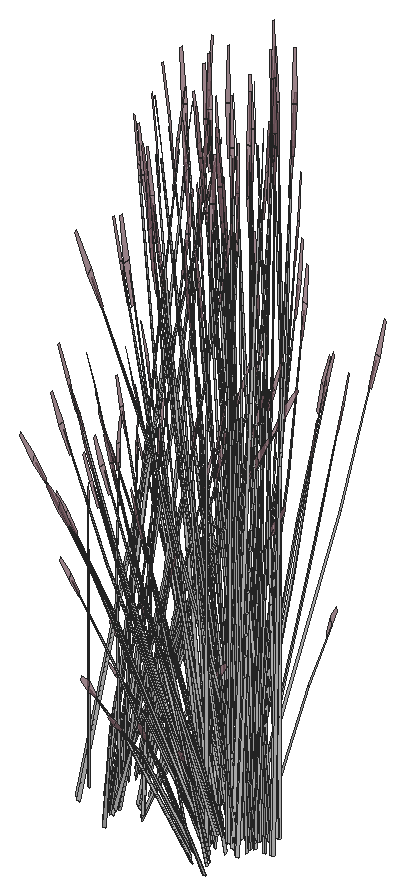
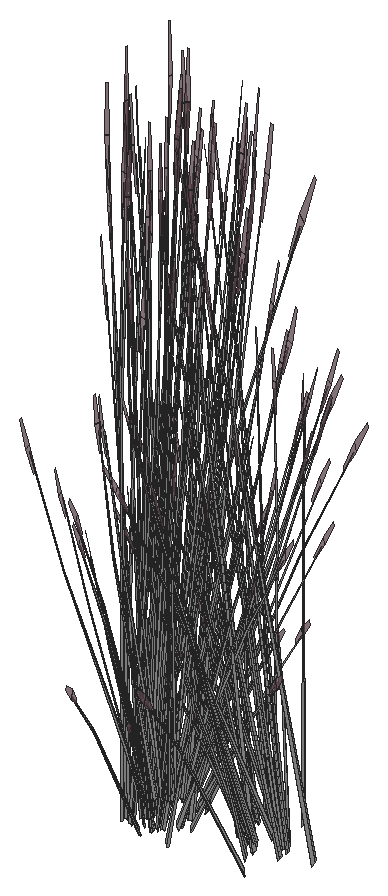
# SketchUp Ruby script. Lengths in inches.
U = 1.inch
M = Sketchup.active_model
def pt(a) = Geom::Point3d.new(a.map { |v| v * U })
def face(e, loops, mat)
  f = e.add_face(loops[0].map { |a| pt(a) })
  loops[1..].each { |l| e.add_face(l.map { |a| pt(a) }).erase! }
  f.material = f.back_material = mat if mat
  f
end
# faces: each face lists its corners as indices into pts; further lists are holes
def faces(e, pts, list, mat = nil) = list.each { |f| face(e, (f[0].is_a?(Array) ? f : [f]).map { |l| l.map { |i| pts[i] } }, mat) }
# xy, xz, yz: faces in a plane at the given z, y or x. An outline is a flat list of corners, or four numbers for a rectangle; further outlines are holes
def ring(l) = l.size == 4 ? [[l[0], l[1]], [l[2], l[1]], [l[2], l[3]], [l[0], l[3]]] : l.each_slice(2).to_a
def flat(e, list, mat, &to3) = list.each { |f| face(e, (f[0].is_a?(Array) ? f : [f]).map { |l| ring(l).map { |u, v| to3.(u, v) } }, mat) }
def xy(e, z, list, mat = nil) = flat(e, list, mat) { |x, y| [x, y, z] }
def xz(e, y, list, mat = nil) = flat(e, list, mat) { |x, z| [x, y, z] }
def yz(e, x, list, mat = nil) = flat(e, list, mat) { |y, z| [x, y, z] }
def lines(e, pts, list) = list.each { |a, b| e.add_line(pt(pts[a]), pt(pts[b])) }
# prism: a flat outline (further loops are holes) pulled along v
def prism(e, loops, v, mat = nil)
  f = face(e, loops, mat); d = Geom::Vector3d.new(v.map { |x| x * U })
  f.pushpull(f.normal.samedirection?(d) ? d.length : -d.length)
end
def box(e, o, s, mat = nil) = prism(e, [[o, [o[0] + s[0], o[1], o[2]], [o[0] + s[0], o[1] + s[1], o[2]], [o[0], o[1] + s[1], o[2]]]], [0, 0, s[2]], mat)
def at(x, y, z, deg = 0) = Geom::Transformation.translation(pt([x, y, z])) * Geom::Transformation.rotation(ORIGIN, Z_AXIS, deg.degrees)
def axes(o, x, y, z) = Geom::Transformation.new([*x, 0, *y, 0, *z, 0, *pt(o).to_a, 1])
def part(name) = M.definitions.add(name)
# library, detail: a bought-in or finely detailed component or shape, given as its bounding box
def library(name, o, s) = part(name).tap { |d| box(d.entities, o, s) }
def detail(e, o, s) = box(e.add_group.entities, o, s)
def put(e, d, t, mat = nil) = e.add_instance(d, t).tap { |i| i.material = mat if mat }
def group(e, t, mat = nil) = e.add_group.tap { |g| g.transformation = t; g.material = mat if mat }.entities
root = M.entities
M.materials.add("LightPink_Translucent").color = [144, 107, 117]
M.materials["LightPink_Translucent"].alpha = 0.75
M.materials.add("[_0053_Ivory_]").color = [200, 200, 200]
c1 = part("blade")
p = [[2.15,0.21,22],[0,0.17,0],[0.09,0.45,0],[2.18,0.31,22],[2.29,0.31,22],[0.38,0.45,0],
  [2.48,0.24,33],[2.49,0.24,33],[2.48,0.22,33]]
faces(c1.entities,p,[[0,1,2,3],[4,5,2,3],[6,3,4,7],[8,0,3,6]])
c2 = part("seeds")
p = [[0.3,-0.1,1.38],[-0.01,-0.03,1.59],[-0.01,-0.03,0.03],[0.14,-0.07,-0.07],[0.29,-0.03,3],[0.15,0.01,3.11]]
faces(c2.entities,p,[[0,1,2,3],[1,0,4,5]],"LightPink_Translucent")
c3 = part("blade with seeds")
put(c3.entities,c1,at(0,0,0))
put(c3.entities,c2,axes([2.4,0.25,30.99],[1.5799,-0.05474,1.17369],[-0.12525,1.92788,0.29478],[-0.07173,-0.02425,1.56792]))
put(root,c3,axes([430.06,98.57,130.53],[0.21074,-0.13302,1.71376],[0.17741,0.61464,0.13857],[-0.33083,0.13891,0.73262]),"[_0053_Ivory_]")
put(root,c3,axes([429.4,99.62,129.24],[0.21107,0.05162,1.43002],[0.13604,0.52729,-0.30754],[-0.28671,0.0987,0.61141]),"[_0053_Ivory_]")
put(root,c3,axes([422.4,96.86,128.68],[0.14267,0.54795,-0.30978],[-0.56663,0.1556,0.30978],[0.11423,0.06319,1.38974]),"[_0053_Ivory_]")
put(root,c3,axes([423.47,98.64,129.03],[0.75945,0,0],[0,0.70283,-0.51607],[0,0.16007,1.63711]),"[_0053_Ivory_]")
put(root,c3,axes([421.01,97.73,129.32],[0.61322,-0.4175,-0.29095],[0.40778,0.58992,-0.50002],[0.1513,0.05991,1.59708]),"[_0053_Ivory_]")
put(root,c3,axes([431.27,97.93,130],[0.17264,-0.09097,1.77064],[0.05953,0.63516,0.13857],[-0.37394,0.08428,0.63284]),"[_0053_Ivory_]")
put(root,c3,axes([422.49,101.25,129.32],[-0.38947,-0.01972,1.0506],[0.25721,-0.41888,0.58006],[0.15386,0.14882,0.8241]),"[_0053_Ivory_]")
put(root,c3,axes([421.3125,96.22,130.53],[-0.11309,0.21615,1.71376],[-0.47441,-0.44731,0.13857],[0.21402,-0.27879,0.73262]),"[_0053_Ivory_]")
put(root,c3,axes([430.71,96.91,131.63],[-0.60713,-0.01514,-0.71045],[0.04078,-0.63759,0.08574],[-0.25721,-0.06729,1.00501]),"[_0053_Ivory_]")
put(root,c3,axes([419.47,97.36,128.25],[-0.59782,0.25177,1.28929],[-0.19028,-0.72239,0.50096],[0.36709,0.01202,1.46642]),"[_0053_Ivory_]")
put(root,c3,axes([430.22,97.07,129.24],[0.11858,0.17508,1.43002],[-0.27325,0.4759,-0.30754],[-0.28057,-0.11375,0.61141]),"[_0053_Ivory_]")
put(root,c3,axes([429.73,98.02,131.18],[-0.50475,-0.17543,-0.35414],[0.14722,-0.5118,0.4572],[-0.20322,0.04693,0.87481]),"[_0053_Ivory_]")
put(root,c3,axes([430.43,96.5,130.53],[0.2256,0.10835,1.71376],[-0.46687,0.45453,0.13857],[-0.29098,-0.20505,0.73262]),"[_0053_Ivory_]")
put(root,c3,axes([421.66,100.67,131.33],[0.59932,-0.14948,-0.51099],[0.10484,0.56611,-0.3958],[0.16097,0.16223,0.97773]),"[_0053_Ivory_]")
put(root,c3,axes([422.21,96.24,129.03],[0.37973,-0.63014,0],[0.6353,0.35142,-0.51607],[0.14469,0.08004,1.63711]),"[_0053_Ivory_]")
put(root,c3,axes([422.85,95.97,128.15],[-0.0909,-0.04954,1.76342],[-0.2335,-0.55347,-0.26939],[0.15752,-0.1502,0.30037]),"[_0053_Ivory_]")
put(root,c3,axes([430.08,98.28,131.33],[-0.16454,0.57202,-0.51099],[-0.56413,-0.19607,-0.3958],[-0.22713,0.05245,0.97773]),"[_0053_Ivory_]")
put(root,c3,axes([422.56,96.62,128.67],[0.56842,0.31443,-0.49651],[-0.33976,0.56381,0],[0.12946,0.07161,1.57504]),"[_0053_Ivory_]")
put(root,c3,axes([430.51,97.04,131.33],[-0.44101,0.41656,-0.51099],[-0.38623,-0.44004,-0.3958],[-0.22407,-0.06338,0.97773]),"[_0053_Ivory_]")
put(root,c3,axes([429.8,98.24,128.15],[0.0154,0.09911,1.76342],[-0.31051,0.51756,-0.26939],[-0.22056,-0.02609,0.30037]),"[_0053_Ivory_]")
put(root,c3,axes([422.53,101.1,128.15],[0.04425,-0.09079,1.76342],[0.55709,-0.26738,-0.26939],[0.16889,0.13839,0.30037]),"[_0053_Ivory_]")
put(root,c3,axes([422.83,97.3,131.33],[-0.15602,-0.5742,-0.51099],[0.59087,-0.10045,-0.3958],[0.16933,-0.15423,0.97773]),"[_0053_Ivory_]")
put(root,c3,axes([423.87,100.26,130.58],[-0.11624,-0.52862,-0.03492],[0.54943,-0.12153,-0.15832],[0.11473,0.03351,0.52218]),"[_0053_Ivory_]")
put(root,c3,axes([421.73,97.83,128.71],[0.63179,0.1031,-0.62353],[-0.13332,0.63596,-0.16365],[0.18854,0.07706,1.37633]),"[_0053_Ivory_]")
put(root,c3,axes([428.96,100.73,129.42],[0.25312,-0.28501,1.1486],[0.09988,0.45119,0.84392],[-0.18292,0.08079,0.25299]),"[_0053_Ivory_]")
put(root,c3,axes([424.42,98.2,128.91],[-0.37654,-0.40212,-0.06488],[0.4124,-0.36845,-0.29416],[0.11685,-0.02594,0.97024]),"[_0053_Ivory_]")
put(root,c3,axes([423.56,96.15,129.42],[-0.2023,0.32011,1.1486],[-0.17388,-0.43009,0.84392],[0.16708,-0.10777,0.25299]),"[_0053_Ivory_]")
put(root,c3,axes([430.34,96.65,131.18],[-0.34557,-0.39372,-0.35414],[0.39459,-0.37271,0.4572],[-0.20048,-0.05671,0.87481]),"[_0053_Ivory_]")
put(root,c3,axes([430.83,98.99,130.53],[0.1517,-0.19322,1.71376],[0.38303,0.52154,0.13857],[-0.26271,0.23751,0.73262]),"[_0053_Ivory_]")
put(root,c3,axes([429.92,99.49,131.18],[-0.52868,0.08987,-0.35414],[-0.1396,-0.51376,0.4572],[-0.1515,0.13799,0.87481]),"[_0053_Ivory_]")
put(root,c3,axes([429.63,101.02,128.15],[0.08147,0.06283,1.76342],[0.13814,0.58211,-0.26939],[-0.18056,0.12413,0.30037]),"[_0053_Ivory_]")
put(root,c3,axes([429.51,97.59,129.42],[0.38775,-0.045,1.1486],[-0.24596,0.39648,0.84392],[-0.19161,-0.05948,0.25299]),"[_0053_Ivory_]")
put(root,c3,axes([421.6,99.19,130.53],[-0.2256,-0.10835,1.71376],[0.46687,-0.45453,0.13857],[0.29098,0.20505,0.73262]),"[_0053_Ivory_]")
put(root,c3,axes([423.27,97.36,131.18],[0.52868,-0.08987,-0.35414],[0.1396,0.51376,0.4572],[0.1515,-0.13799,0.87481]),"[_0053_Ivory_]")
put(root,c3,axes([422.85,97.53,131.63],[0.31725,-0.49618,-0.71045],[0.55593,0.35263,0.08574],[0.18942,-0.17977,1.00501]),"[_0053_Ivory_]")
put(root,c3,axes([422.84,100.2,131.18],[0.34557,0.39372,-0.35414],[-0.39459,0.37271,0.4572],[0.20048,0.05671,0.87481]),"[_0053_Ivory_]")
put(root,c3,axes([430.72,99.46,130.53],[0.11309,-0.21615,1.71376],[0.47441,0.44731,0.13857],[-0.21402,0.27879,0.73262]),"[_0053_Ivory_]")
put(root,c3,axes([430.35,99.55,131.33],[0.15602,0.5742,-0.51099],[-0.59087,0.10045,-0.3958],[-0.16933,0.15423,0.97773]),"[_0053_Ivory_]")
put(root,c3,axes([431.83,99.14,128.71],[-0.63179,-0.1031,-0.62353],[0.13332,-0.63596,-0.16365],[-0.18854,-0.07706,1.37633]),"[_0053_Ivory_]")
put(root,c3,axes([423.11,98.57,131.33],[0.16454,-0.57202,-0.51099],[0.56413,0.19607,-0.3958],[0.22713,-0.05245,0.97773]),"[_0053_Ivory_]")
put(root,c3,axes([424.52,98.9375,129.42],[-0.37526,0.10382,1.1486],[0.17664,-0.42906,0.84392],[0.19907,0.02936,0.25299]),"[_0053_Ivory_]")
put(root,c3,axes([431.76,96.16,131.63],[-0.51789,-0.30395,-0.71045],[0.36805,-0.53263,0.08574],[-0.18764,-0.18149,1.00501]),"[_0053_Ivory_]")
put(root,c3,axes([431.52,96.18,131.33],[-0.59932,0.14948,-0.51099],[-0.10484,-0.56611,-0.3958],[-0.16097,-0.16223,0.97773]),"[_0053_Ivory_]")
put(root,c3,axes([423.31,97.07,129.24],[-0.21697,-0.01863,1.43002],[-0.22228,-0.49966,-0.30754],[0.26655,-0.14135,0.61141]),"[_0053_Ivory_]")
put(root,c3,axes([423.45,98.83,131.18],[0.50475,0.17543,-0.35414],[-0.14722,0.5118,0.4572],[0.20322,-0.04693,0.87481]),"[_0053_Ivory_]")
put(root,c3,axes([431,100.34,128.67],[-0.56842,-0.31443,-0.49651],[0.33976,-0.56381,0],[-0.12946,-0.07161,1.57504]),"[_0053_Ivory_]")
put(root,c3,axes([430.75,95.66,128.15],[-0.05883,0.08284,1.76342],[-0.59454,0.17861,-0.26939],[-0.14363,-0.16248,0.30037]),"[_0053_Ivory_]")
put(root,c3,axes([422.48,99.9375,131.63],[0.60713,0.01514,-0.71045],[-0.04078,0.63759,0.08574],[0.25721,0.06729,1.00501]),"[_0053_Ivory_]")
put(root,c3,axes([431.34,100.72,129.03],[-0.37973,0.63014,0],[-0.6353,-0.35142,-0.51607],[-0.14469,-0.08004,1.63711]),"[_0053_Ivory_]")
put(root,c3,axes([423.71,98.73,128.64],[-0.39118,0.07547,1.41583],[-0.06226,-0.6007,0.08104],[0.27398,-0.09092,0.80566]),"[_0053_Ivory_]")
put(root,c3,axes([424.14,98.34,128.15],[-0.03174,-0.09547,1.76342],[0.22015,-0.55846,-0.26939],[0.22208,-0.00803,0.30037]),"[_0053_Ivory_]")
put(root,c3,axes([422.08,98.2,130.53],[-0.25192,0.01424,1.71376],[0.16712,-0.61729,0.13857],[0.35901,0.03818,0.73262]),"[_0053_Ivory_]")
put(root,c3,axes([430.65,101.64,129.24],[0.19166,-0.0992,1.43002],[0.4732,0.29912,-0.30754],[-0.14084,0.25882,0.61141]),"[_0053_Ivory_]")
put(root,c3,axes([423,98.78,131.63],[0.53369,-0.27773,-0.71045],[0.29743,0.5717,0.08574],[0.25786,-0.06494,1.00501]),"[_0053_Ivory_]")
put(root,c3,axes([430.38,95.98,128.78],[-0.1752,0.51349,-0.03893],[-0.53924,-0.15795,-0.17649],[-0.08187,-0.08399,0.58215]),"[_0053_Ivory_]")
put(root,c3,axes([431.18,95.33,129.24],[-0.03678,0.20572,1.43002],[-0.53767,0.17221,-0.30754],[-0.12568,-0.26589,0.61141]),"[_0053_Ivory_]")
put(root,c3,axes([431.36,95.87,130.53],[0.13883,0.2019,1.71376],[-0.64153,0.16998,0.13857],[-0.14499,-0.31697,0.73262]),"[_0053_Ivory_]")
put(root,c3,axes([432.54,99.24,129.32],[-0.61322,0.4175,-0.29095],[-0.40778,-0.58992,-0.50002],[-0.1513,-0.05991,1.59708]),"[_0053_Ivory_]")
put(root,c3,axes([431.58,95.76,131.18],[-0.0938,-0.50652,-0.35414],[0.53623,-0.13375,0.4572],[-0.14403,-0.14515,0.87481]),"[_0053_Ivory_]")
put(root,c3,axes([430.09,98.32,129.03],[-0.75945,0,0],[0,-0.70283,-0.51607],[0,-0.16007,1.63711]),"[_0053_Ivory_]")
put(root,c3,axes([431.16,100.11,128.68],[-0.14267,-0.54795,-0.30978],[0.56663,-0.1556,0.30978],[-0.11423,-0.06319,1.38974]),"[_0053_Ivory_]")
put(root,c3,axes([423.82,99.625,129.24],[-0.14627,-0.15466,1.43002],[0.19032,-0.51164,-0.30754],[0.29594,0.06931,0.61141]),"[_0053_Ivory_]")
put(root,c3,axes([430.85,100.68,131.18],[-0.41095,0.33109,-0.35414],[-0.38901,-0.37805,0.4572],[-0.05919,0.19208,0.87481]),"[_0053_Ivory_]")
put(root,c3,axes([432.95,99.69,128.71],[-0.40909,0.47266,-0.62353],[-0.50819,-0.4286,-0.16365],[-0.16393,0.11791,1.37633]),"[_0053_Ivory_]")
put(root,c3,axes([430.68,98.14,128.98],[-0.56493,0.5287,0.30756],[-0.56528,-0.52313,-0.36492],[-0.01973,-0.15014,1.64885]),"[_0053_Ivory_]")
put(root,c3,axes([433,99.6,129.98],[0.52485,0.25358,1.51261],[-0.51417,0.54629,0.59816],[-0.23031,-0.32378,1.26806]),"[_0053_Ivory_]")
put(root,c3,axes([431,95,129.42],[0.31682,0.21887,1.1486],[-0.4614,0.13157,0.84392],[-0.09872,-0.16821,0.25299]),"[_0053_Ivory_]")
put(root,c3,axes([433.23,99.43,129.12],[-0.59306,-0.50614,-0.25192],[0.49904,-0.56836,0.5513],[-0.1597,0.05921,1.68216]),"[_0053_Ivory_]")
put(root,c3,axes([432.15,98.9375,128.86],[-0.36485,-0.52782,-0.44739],[0.55265,-0.37168,0.21531],[-0.11807,-0.06531,1.43643]),"[_0053_Ivory_]")
put(root,c3,axes([431.12,100.33,131.99],[-0.0158,0.58168,-0.7886],[-0.66548,-0.03907,0.09517],[-0.07023,0.24643,1.11556]),"[_0053_Ivory_]")
put(root,c3,axes([431.11,101.97,129.42],[-0.01572,-0.37392,1.1486],[0.39276,0.26669,0.84392],[-0.07724,0.17822,0.25299]),"[_0053_Ivory_]")
put(root,c3,axes([432.93,99.32,128.86],[-0.65953,0.03882,-0.44739],[-0.05964,-0.64439,0.21531],[-0.11807,0.06531,1.43643]),"[_0053_Ivory_]")
put(root,c3,axes([431.67,100.4,129.13],[0.56842,0.31443,0.49651],[-0.33976,0.56381,0],[-0.12946,-0.07161,1.57504]),"[_0053_Ivory_]")
put(root,c3,axes([430.9,101.15,130.02],[0.01334,-0.32463,1.54345],[0.60018,0.17147,0.21329],[-0.052,0.34598,0.72882]),"[_0053_Ivory_]")
put(root,c3,axes([432.21,99.24,129.09],[0.16098,-0.74515,-0.23429],[0.76326,0.12989,0.51271],[-0.13337,-0.1029,1.5644]),"[_0053_Ivory_]")
put(root,c3,axes([432.49,99.42,129.27],[-0.11717,0.56122,0.1448],[-0.57245,-0.09742,-0.41347],[-0.10418,-0.05763,1.26744]),"[_0053_Ivory_]")
put(root,c3,axes([433.625,100.98,128.67],[-0.56842,0.31443,-0.49651],[-0.33976,-0.56381,0],[-0.12946,0.07161,1.57504]),"[_0053_Ivory_]")
put(root,c3,axes([430.26,97.85,128.67],[0,-0.62885,-0.49651],[0.67951,0,0],[0,-0.14322,1.57504]),"[_0053_Ivory_]")
put(root,c3,axes([430.55,98.43,129.13],[0,0.62885,0.49651],[-0.67951,0,0],[0,-0.14322,1.57504]),"[_0053_Ivory_]")
put(root,c3,axes([433.66,100.8125,128.85],[-0.37499,-0.63235,-0.05142],[0.6353,-0.35142,0.51607],[-0.15655,0.0602,1.6363]),"[_0053_Ivory_]")
put(root,c3,axes([431.26,100.53,131.66],[0.43478,0.42253,-0.5672],[-0.45929,0.37004,-0.43934],[-0.06615,0.21468,1.08528]),"[_0053_Ivory_]")
put(root,c3,axes([433.49,100.73,128.68],[-0.56663,-0.1556,-0.30978],[0.14267,-0.54795,0.30978],[-0.11423,0.06319,1.38974]),"[_0053_Ivory_]")
put(root,c3,axes([432.04,98.58,129.32],[-0.68399,-0.30005,-0.29095],[0.32934,-0.63331,-0.50002],[-0.0215,-0.15549,1.59708]),"[_0053_Ivory_]")
put(root,c3,axes([433.82,98.39,129.5],[-0.01659,-0.59209,1.41272],[0.75089,0.15348,0.59816],[-0.1776,0.32398,1.3335]),"[_0053_Ivory_]")
put(root,c3,axes([430.78,101.16,129.48],[0.55175,-0.11136,0.06507],[0.12684,0.44864,-0.86304],[-0.03498,0.22711,0.7736]),"[_0053_Ivory_]")
put(root,c3,axes([433.39,99.14,129.32],[0.07077,0.71755,-0.29095],[-0.73712,0.04339,-0.50002],[-0.1298,0.09558,1.59708]),"[_0053_Ivory_]")
put(root,c3,axes([431.73,97.9375,128.75],[-0.24943,-0.64486,-0.69835],[0.71849,-0.23224,-0.18329],[-0.02757,-0.21836,1.54149]),"[_0053_Ivory_]")
put(root,c3,axes([432.85,95.91,131.33],[-0.59704,-0.15764,-0.51099],[0.20464,-0.54049,-0.3958],[-0.05475,-0.21761,0.97773]),"[_0053_Ivory_]")
put(root,c3,axes([431.75,99.92,130.53],[-0.01487,-0.24136,1.71376],[0.64429,0.16012,0.13857],[-0.03985,0.34396,0.73262]),"[_0053_Ivory_]")
put(root,c3,axes([430.55,97.86,128.68],[0.42396,-0.39235,-0.30978],[0.42396,0.39235,0.30978],[0,-0.12637,1.38974]),"[_0053_Ivory_]")
put(root,c3,axes([432.47,95.32,128.78],[-0.4197,0.36076,-0.03893],[-0.38456,-0.39511,-0.17649],[-0.02707,-0.11196,0.58215]),"[_0053_Ivory_]")
put(root,c3,axes([432.3,98.88,129.01],[0.76764,0.13249,0.45755],[-0.15622,0.74829,0.17955],[-0.11218,-0.07226,1.58856]),"[_0053_Ivory_]")
put(root,c3,axes([432.1,98.75,129.37],[-0.29468,0.56664,0.44739],[-0.61229,-0.27271,-0.21531],[0,-0.13062,1.43643]),"[_0053_Ivory_]")
put(root,c3,axes([433.07,96.02,131.63],[-0.28988,-0.51132,-0.71045],[0.59671,-0.28496,0.08574],[-0.06778,-0.24706,1.00501]),"[_0053_Ivory_]")
put(root,c3,axes([431.88,100.08,129.13],[0.65264,-0.16691,0.17642],[0.16115,0.62115,0.35086],[-0.05821,-0.0905,1.60407]),"[_0053_Ivory_]")
put(root,c3,axes([432.72,100.18,128.85],[-0.61229,-0.28233,0],[0.29468,-0.58663,0],[0,0,1.62707]),"[_0053_Ivory_]")
put(root,c3,axes([434.14,100.88,129.03],[0.37973,0.63014,0],[-0.6353,0.35142,-0.51607],[-0.14469,0.08004,1.63711]),"[_0053_Ivory_]")
put(root,c3,axes([433.83,100.11,129.13],[0.17545,-0.62497,0.17642],[0.64204,0.17686,0.35086],[-0.11091,0.00304,1.60407]),"[_0053_Ivory_]")
put(root,c3,axes([433.53,99.28,129.27],[0.44871,0.37783,0.1448],[-0.37428,0.42627,-0.41347],[-0.10418,0.05763,1.26744]),"[_0053_Ivory_]")
put(root,c3,axes([433.37,98.82,128.95],[-0.56493,-0.54126,-0.06131],[0.56528,-0.54159,0],[-0.01973,-0.0189,1.75571]),"[_0053_Ivory_]")
put(root,c3,axes([433.52,99.01,129.37],[0.65953,-0.03882,0.44739],[0.05964,0.64439,-0.21531],[-0.11807,0.06531,1.43643]),"[_0053_Ivory_]")
put(root,c3,axes([433.68,100.49,128.98],[0.76036,0.2044,0.30756],[-0.19023,0.7306,-0.36492],[-0.12585,0.09144,1.64885]),"[_0053_Ivory_]")
put(root,c3,axes([432.57,94.88,128.15],[-0.10187,0.02266,1.76342],[-0.56336,-0.25503,-0.26939],[0.00945,-0.21273,0.30037]),"[_0053_Ivory_]")
put(root,c3,axes([434.01,100.45,129.13],[0.56842,-0.31443,0.49651],[0.33976,0.56381,0],[-0.12946,0.07161,1.57504]),"[_0053_Ivory_]")
put(root,c3,axes([433.125,95.58,131.18],[0.1831,-0.48359,-0.35414],[0.53419,0.14105,0.4572],[-0.04898,-0.1947,0.87481]),"[_0053_Ivory_]")
put(root,c3,axes([432.23,98.19,129.01],[0.26406,0.70318,0.45755],[-0.7545,0.24452,0.17955],[0.00922,-0.12921,1.58856]),"[_0053_Ivory_]")
put(root,c3,axes([432.11,98.1,128.86],[0.29468,-0.56664,-0.44739],[0.61229,0.27271,0.21531],[0,-0.13062,1.43643]),"[_0053_Ivory_]")
put(root,c3,axes([432.86,99.93,128.86],[-0.19817,-0.54216,0],[0.56587,-0.18986,0],[0,0,1.54371]),"[_0053_Ivory_]")
put(root,c3,axes([432.14,101.08,128.15],[0.09829,-0.03422,1.76342],[0.59126,0.18834,-0.26939],[0.01729,0.21228,0.30037]),"[_0053_Ivory_]")
put(root,c3,axes([432.27,101.27,131.18],[-0.1831,0.48359,-0.35414],[-0.53419,-0.14105,0.4572],[0.04898,0.1947,0.87481]),"[_0053_Ivory_]")
put(root,c3,axes([433.66,98.86,128.86],[-0.29468,0.56664,-0.44739],[-0.61229,-0.27271,0.21531],[0,0.13062,1.43643]),"[_0053_Ivory_]")
put(root,c3,axes([434.83,98.52,129.13],[-0.47719,-0.45806,0.17642],[0.48088,-0.44429,0.35086],[-0.0527,0.09355,1.60407]),"[_0053_Ivory_]")
put(root,c3,axes([433.18,98.25,128.86],[0,-0.72763,0],[0.75945,0,0],[0,0,1.79456]),"[_0053_Ivory_]")
put(root,c3,axes([432.47,98.39,129.09],[0.68433,0.30479,0.24065],[-0.32934,0.63331,0.50002],[0,-0.14599,1.60543]),"[_0053_Ivory_]")
put(root,c3,axes([433.5625,98.54,128.95],[0,0.72727,-0.05637],[-0.75945,0,0],[0,0.02286,1.79368]),"[_0053_Ivory_]")
put(root,c3,axes([432.25,97.96,129.37],[-0.65953,0.03882,0.44739],[-0.05964,-0.64439,-0.21531],[0.11807,-0.06531,1.43643]),"[_0053_Ivory_]")
put(root,c3,axes([431.95,96.85,129.13],[-0.17545,0.62497,0.17642],[-0.64204,-0.17686,0.35086],[0.11091,-0.00304,1.60407]),"[_0053_Ivory_]")
put(root,c3,axes([433.2,99.95,128.94],[0.26406,0.72244,-0.06012],[-0.7545,0.25315,0],[0.00922,0.02523,1.72173]),"[_0053_Ivory_]")
put(root,c3,axes([431.63,96.08,129.03],[-0.37973,-0.63014,0],[0.6353,-0.35142,-0.51607],[0.14469,-0.08004,1.63711]),"[_0053_Ivory_]")
put(root,c3,axes([432.33,100.83,131.63],[0.28988,0.51132,-0.71045],[-0.59671,0.28496,0.08574],[0.06778,0.24706,1.00501]),"[_0053_Ivory_]")
put(root,c3,axes([435.38,99,128.85],[-0.75908,-0.00503,-0.04976],[0,-0.70283,0.49943],[-0.02386,0.16,1.58352]),"[_0053_Ivory_]")
put(root,c3,axes([433.89,96.89,129.13],[-0.65264,0.16691,0.17642],[-0.16115,-0.62115,0.35086],[0.05821,0.0905,1.60407]),"[_0053_Ivory_]")
put(root,c3,axes([433.22,94.5625,129.42],[0.07791,0.3667,1.1486],[-0.43222,-0.2031,0.84392],[0.04651,-0.18776,0.25299]),"[_0053_Ivory_]")
put(root,c3,axes([432.82,97.79,129.01],[-0.50358,0.57069,0.45755],[-0.59827,-0.50377,0.17955],[0.1214,-0.05695,1.58856]),"[_0053_Ivory_]")
put(root,c3,axes([433.68,98.69,128.87],[0.42396,0.40619,0],[-0.42396,0.40619,0],[0,0,1.69266]),"[_0053_Ivory_]")
